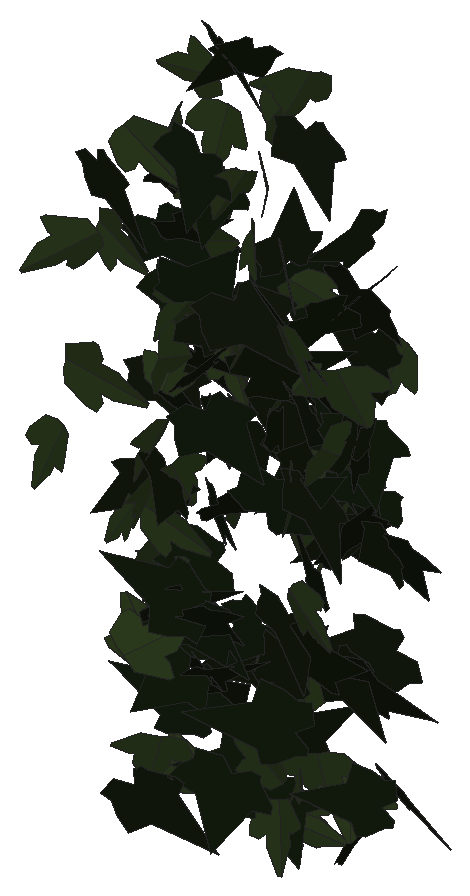
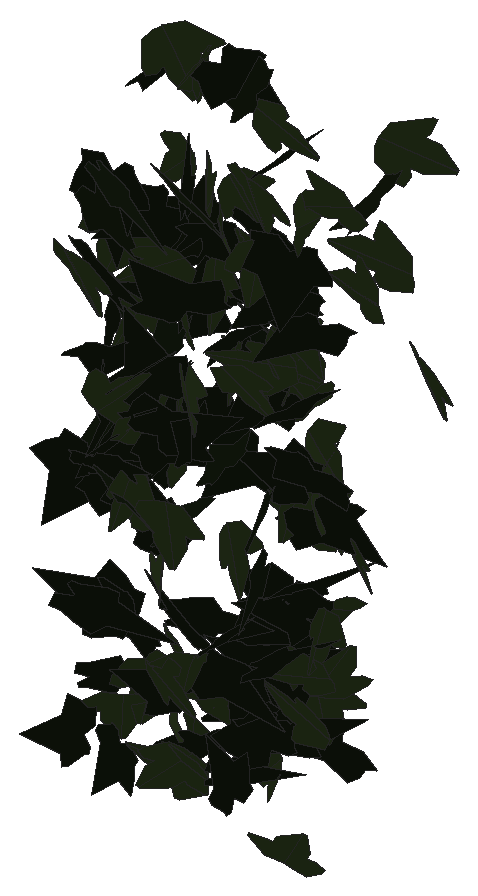
# SketchUp Ruby script. Lengths in inches.
U = 1.inch
M = Sketchup.active_model
def pt(a) = Geom::Point3d.new(a.map { |v| v * U })
def face(e, loops, mat)
  f = e.add_face(loops[0].map { |a| pt(a) })
  loops[1..].each { |l| e.add_face(l.map { |a| pt(a) }).erase! }
  f.material = f.back_material = mat if mat
  f
end
# faces: each face lists its corners as indices into pts; further lists are holes
def faces(e, pts, list, mat = nil) = list.each { |f| face(e, (f[0].is_a?(Array) ? f : [f]).map { |l| l.map { |i| pts[i] } }, mat) }
# xy, xz, yz: faces in a plane at the given z, y or x. An outline is a flat list of corners, or four numbers for a rectangle; further outlines are holes
def ring(l) = l.size == 4 ? [[l[0], l[1]], [l[2], l[1]], [l[2], l[3]], [l[0], l[3]]] : l.each_slice(2).to_a
def flat(e, list, mat, &to3) = list.each { |f| face(e, (f[0].is_a?(Array) ? f : [f]).map { |l| ring(l).map { |u, v| to3.(u, v) } }, mat) }
def xy(e, z, list, mat = nil) = flat(e, list, mat) { |x, y| [x, y, z] }
def xz(e, y, list, mat = nil) = flat(e, list, mat) { |x, z| [x, y, z] }
def yz(e, x, list, mat = nil) = flat(e, list, mat) { |y, z| [x, y, z] }
def lines(e, pts, list) = list.each { |a, b| e.add_line(pt(pts[a]), pt(pts[b])) }
# prism: a flat outline (further loops are holes) pulled along v
def prism(e, loops, v, mat = nil)
  f = face(e, loops, mat); d = Geom::Vector3d.new(v.map { |x| x * U })
  f.pushpull(f.normal.samedirection?(d) ? d.length : -d.length)
end
def box(e, o, s, mat = nil) = prism(e, [[o, [o[0] + s[0], o[1], o[2]], [o[0] + s[0], o[1] + s[1], o[2]], [o[0], o[1] + s[1], o[2]]]], [0, 0, s[2]], mat)
def at(x, y, z, deg = 0) = Geom::Transformation.translation(pt([x, y, z])) * Geom::Transformation.rotation(ORIGIN, Z_AXIS, deg.degrees)
def axes(o, x, y, z) = Geom::Transformation.new([*x, 0, *y, 0, *z, 0, *pt(o).to_a, 1])
def part(name) = M.definitions.add(name)
# library, detail: a bought-in or finely detailed component or shape, given as its bounding box
def library(name, o, s) = part(name).tap { |d| box(d.entities, o, s) }
def detail(e, o, s) = box(e.add_group.entities, o, s)
def put(e, d, t, mat = nil) = e.add_instance(d, t).tap { |i| i.material = mat if mat }
def group(e, t, mat = nil) = e.add_group.tap { |g| g.transformation = t; g.material = mat if mat }.entities
root = M.entities
M.materials.add("1026 AP 7946 SUNNY SIDE UP").color = [254, 231, 186]
M.materials.add("efeu1").color = [18, 25, 13]
M.materials.add("efeu2").color = [43, 57, 29]
c1 = part("ivyleaf_10")
p = [[0,0.5,-0.03],[-0.0625,2.02,-0.43],[-0.19,2.01,-0.46],[-0.54,1.05,-0.29],[-0.52,0.625,-0.18],[-0.83,0.76,-0.28],
  [-1.16,0.64,-0.33],[-1.15,0.33,-0.24],[-0.77,-0.39,0.02],[-0.3,-0.51,0.16],[0.04,-0.48,0.23],[-0.02,2.01,-0.4375],
  [-0.06,2.01,-0.43],[0.04,-0.49,0.23],[0.67,-0.49,0.14],[1.38,0.36,-0.2],[1.375,0.51,-0.24],[0.81,0.65,-0.19],
  [0.62,0.59,-0.15],[0.6,1.09,-0.28],[0.5,1.23,-0.31]]
faces(c1.entities,p,[[0,1,2,3,4,5,6,7,8,9,10],[11,12,0,13,14,15,16,17,18,19,20]],"efeu2")
c2 = part("ivyleaf_9")
p = [[1.54,2.16,1.25],[1.36,2.04,1.19],[-0.21,0.99,0.68],[-0.71,1.11,0.82],[-0.85,0.86,0.67],[-0.8,0.17,0.21],
  [-0.9,-0.01,0.1],[-0.67,-0.16,-0.02],[-0.08,-0.08,-0.05],[-0.03,-0.6,-0.4],[0.65,-0.88,-0.66],[0.83,-0.6,-0.49],
  [1.29,-0.42,-0.43],[1.8125,-0.07,-0.26],[1.21,0.44,0.15]]
faces(c2.entities,p,[[0,1,2,3,4,5,6,7,8,9,10,11,12,13,14]],"efeu1")
put(root,c1,axes([128.42,208.2,277.38],[-0.11981,-0.18538,0.35374],[-0.16586,-0.32816,-0.20792],[0.59225,-0.1294,0.01334]),"1026 AP 7946 SUNNY SIDE UP")
put(root,c1,axes([128.52,208.07,275.41],[0.02717,0.00224,0.40839],[0.62094,0.03465,-0.01773],[-0.05458,0.39527,0.00157]),"1026 AP 7946 SUNNY SIDE UP")
put(root,c1,axes([127.97,208.17,274.1],[0.44169,-0.27483,0.02712],[0.00539,-0.0363,-0.40434],[0.43433,0.27994,-0.02256]),"1026 AP 7946 SUNNY SIDE UP")
put(root,c1,axes([131.47,209,276.5],[-0.30463,0.20215,-0.19161],[0.17913,-0.14952,-0.28875],[-0.39439,-0.22405,0.01685]),"1026 AP 7946 SUNNY SIDE UP")
put(root,c2,axes([128.72,209.08,268.42],[0.0398,-0.10331,-0.35879],[0.46844,0.20474,-0.03913],[0.32534,-0.28215,0.10024]),"1026 AP 7946 SUNNY SIDE UP")
put(root,c1,axes([128.98,209.22,269.13],[-0.37267,-0.23168,0.04947],[-0.02963,-0.05113,-0.34091],[0.37129,-0.23663,0.02245]),"1026 AP 7946 SUNNY SIDE UP")
put(root,c1,axes([131.36,209.375,272.16],[-0.19428,0.10101,-0.33264],[0.32312,-0.25144,-0.16322],[-0.4237,-0.23807,0.02805]),"1026 AP 7946 SUNNY SIDE UP")
put(root,c1,axes([128.6,209.1875,270.54],[0.31198,0.0225,-0.31751],[0.3079,0.27435,0.15205],[0.37616,-0.24323,0.13888]),"1026 AP 7946 SUNNY SIDE UP")
put(root,c2,axes([129.91,209.64,268.76],[-0.31064,-0.30865,-0.02061],[0.04185,0.0046,-0.37694],[0.48436,-0.19835,0.01935]),"1026 AP 7946 SUNNY SIDE UP")
put(root,c2,axes([130.95,209.66,269.84],[-0.35005,0.0129,0.30611],[-0.46477,-0.05002,-0.22625],[0.05093,-0.36784,0.03931]),"1026 AP 7946 SUNNY SIDE UP")
put(root,c2,axes([128.98,209.82,270.02],[-0.31738,-0.20262,0.15102],[-0.12374,-0.1289,-0.29362],[0.37439,-0.21437,0.03098]),"1026 AP 7946 SUNNY SIDE UP")
put(root,c2,axes([129.61,209.51,274.45],[0.01083,-0.23233,-0.30337],[0.01332,0.29323,-0.23749],[0.58802,-0.00236,0.01097]),"1026 AP 7946 SUNNY SIDE UP")
put(root,c2,axes([130.75,209.86,271.48],[0.05918,-0.3586,0.16433],[0.0429,-0.15952,-0.37226],[0.61695,0.04549,0.01012]),"1026 AP 7946 SUNNY SIDE UP")
put(root,c1,axes([130.61,209.76,268.36],[0.44483,-0.13392,0.22782],[0.28607,-0.13135,-0.32138],[0.29027,0.33469,-0.0324]),"1026 AP 7946 SUNNY SIDE UP")
put(root,c2,axes([127.52,209.74,277.54],[0.29023,-0.33567,-0.03726],[-0.04253,0.0242,-0.39431],[0.52885,0.18616,-0.01127]),"1026 AP 7946 SUNNY SIDE UP")
put(root,c2,axes([128.56,209.9375,272.9],[-0.02994,-0.24284,0.25414],[-0.02519,-0.24756,-0.25238],[0.54528,-0.02477,0.0023]),"1026 AP 7946 SUNNY SIDE UP")
put(root,c2,axes([131.14,209.77,271.01],[0.06651,-0.0184,0.34077],[0.33948,-0.25154,-0.04431],[0.39534,0.21909,-0.01928]),"1026 AP 7946 SUNNY SIDE UP")
put(root,c2,axes([130.47,209.92,276.11],[0.25901,-0.25402,0.27156],[0.17644,-0.24175,-0.31196],[0.54963,0.19732,-0.02782]),"1026 AP 7946 SUNNY SIDE UP")
put(root,c1,axes([131.83,209.72,275.6875],[-0.48263,-0.23109,-0.12927],[0.1829,0.05141,-0.39449],[0.36973,-0.32708,0.0264]),"1026 AP 7946 SUNNY SIDE UP")
put(root,c2,axes([128.92,209.98,270.99],[-0.18236,-0.36285,-0.08835],[-0.05779,-0.07608,0.39181],[-0.58267,0.12111,-0.01121]),"1026 AP 7946 SUNNY SIDE UP")
put(root,c2,axes([131.43,209.6875,272.125],[0.03109,-0.12438,0.31495],[-0.08241,0.30192,0.1315],[-0.51343,-0.05599,-0.00203]),"1026 AP 7946 SUNNY SIDE UP")
put(root,c1,axes([128.37,209.89,272.25],[0.0374,0.00642,0.39893],[0.60537,-0.04221,-0.02389],[0.06564,0.38563,-0.00697]),"1026 AP 7946 SUNNY SIDE UP")
put(root,c1,axes([128.37,209.97,273.56],[0.06061,-0.34943,0.14222],[0.03445,-0.13845,-0.36292],[0.59092,0.04391,0.00657]),"1026 AP 7946 SUNNY SIDE UP")
put(root,c2,axes([131.04,210.02,273.5],[0.13433,-0.39367,0.03087],[-0.00202,-0.03323,-0.4151],[0.62108,0.08504,-0.00802]),"1026 AP 7946 SUNNY SIDE UP")
put(root,c2,axes([130.51,209.76,273.13],[-0.156,0.06215,0.34462],[0.5213,-0.05907,0.11237],[0.11785,0.34354,-0.04089]),"1026 AP 7946 SUNNY SIDE UP")
put(root,c2,axes([129.91,209.8125,276.16],[0.00295,-0.22583,-0.33937],[0.23158,0.30529,-0.21379],[0.58197,-0.12033,0.08679]),"1026 AP 7946 SUNNY SIDE UP")
put(root,c1,axes([129.15,209.97,268.36],[-0.23781,0.24366,-0.22268],[0.15602,-0.19412,-0.29621],[-0.48934,-0.18031,0.01378]),"1026 AP 7946 SUNNY SIDE UP")
put(root,c1,axes([128.28,209.96,272.72],[0.06747,-0.3707,0.04766],[0.0016,-0.04857,-0.3847],[0.58783,0.04268,-0.00442]),"1026 AP 7946 SUNNY SIDE UP")
put(root,c1,axes([127.86,209.9,272.16],[0.29968,-0.24874,-0.05957],[-0.07734,0.03326,-0.32206],[0.39352,0.19596,-0.01793]),"1026 AP 7946 SUNNY SIDE UP")
put(root,c1,axes([131.58,209.67,274.51],[-0.1065,-0.24369,-0.32412],[0.16029,0.29642,-0.25855],[0.6031,-0.12181,0.01148]),"1026 AP 7946 SUNNY SIDE UP")
put(root,c2,axes([130.55,210.12,276.57],[-0.06709,0.04271,0.32963],[-0.03227,-0.32221,0.03963],[0.50617,-0.01488,0.04621]),"1026 AP 7946 SUNNY SIDE UP")
put(root,c1,axes([130.43,209.84,268.97],[-0.31407,0.0873,-0.30188],[-0.38511,0.16483,0.22316],[0.28905,0.31446,-0.03068]),"1026 AP 7946 SUNNY SIDE UP")
put(root,c2,axes([129.02,209.79,270.9],[0.39646,0.18566,0.07963],[0.116,0.02812,-0.32171],[-0.29349,0.26191,-0.01959]),"1026 AP 7946 SUNNY SIDE UP")
put(root,c2,axes([131.96,209.72,274.51],[0.02494,0.19172,0.28427],[-0.0728,0.27377,-0.19238],[-0.52187,-0.02903,0.04042]),"1026 AP 7946 SUNNY SIDE UP")
put(root,c2,axes([128.85,210.28,277.91],[-0.08492,-0.36305,0.16181],[-0.04475,-0.15664,-0.37902],[0.62169,-0.06086,-0.00518]),"1026 AP 7946 SUNNY SIDE UP")
put(root,c1,axes([127.32,210.14,276.25],[0.07164,-0.00691,0.3717],[0.54256,-0.10579,-0.04759],[0.16637,0.34798,-0.00486]),"1026 AP 7946 SUNNY SIDE UP")
put(root,c2,axes([129.61,209.8,272.9],[0.25531,0.23186,0.16524],[0.15503,0.12509,-0.29076],[-0.41407,0.1898,-0.00697]),"1026 AP 7946 SUNNY SIDE UP")
put(root,c1,axes([130.82,209.84,273.43],[0.10121,-0.21071,-0.34123],[-0.04697,0.33085,-0.22167],[0.6139,0.06005,0.0393]),"1026 AP 7946 SUNNY SIDE UP")
put(root,c2,axes([132.04,210.24,268.78],[-0.25759,-0.02385,0.27858],[-0.39344,-0.10962,-0.16668],[0.16608,-0.29668,0.0372]),"1026 AP 7946 SUNNY SIDE UP")
put(root,c2,axes([128.83,210,274.47],[0.13185,0.30143,0.07099],[-0.04864,-0.06108,0.32168],[0.48316,-0.08841,0.01301]),"1026 AP 7946 SUNNY SIDE UP")
put(root,c2,axes([130.25,210.16,268.44],[-0.11094,-0.29457,-0.15821],[0.0837,0.14322,-0.31075],[0.51438,-0.08684,0.01644]),"1026 AP 7946 SUNNY SIDE UP")
put(root,c2,axes([128.2,210.23,272.65],[0.05694,0.06394,-0.33216],[-0.16625,-0.30526,-0.0763],[-0.48999,0.111,-0.01271]),"1026 AP 7946 SUNNY SIDE UP")
put(root,c2,axes([128.91,209.96,269.75],[0.21284,0.26955,-0.12498],[0.06576,0.11632,0.3111],[0.46112,-0.14101,0.01332]),"1026 AP 7946 SUNNY SIDE UP")
put(root,c2,axes([128.74,210.08,270.77],[-0.09104,-0.11814,-0.3254],[0.308,0.24827,-0.13148],[0.43044,-0.20264,0.02525]),"1026 AP 7946 SUNNY SIDE UP")
put(root,c2,axes([128.39,209.93,270.82],[0.12708,0.22605,-0.22191],[0.06301,0.21449,0.24715],[0.48832,-0.0865,0.02586]),"1026 AP 7946 SUNNY SIDE UP")
put(root,c1,axes([130.05,210.05,275.62],[-0.0313,-0.33319,-0.18832],[0.03506,0.17982,-0.34265],[0.59512,-0.02812,0.01028]),"1026 AP 7946 SUNNY SIDE UP")
put(root,c2,axes([131.875,209.99,274.52],[0.10229,-0.08754,-0.32671],[-0.38917,0.19919,-0.10795],[0.33967,0.25458,-0.0253]),"1026 AP 7946 SUNNY SIDE UP")
put(root,c2,axes([130.12,209.93,275.04],[0.1016,0.06476,0.40098],[0.57149,0.14282,-0.08588],[-0.24006,0.36741,-0.03475]),"1026 AP 7946 SUNNY SIDE UP")
put(root,c1,axes([128.13,210.15,269.94],[0.27018,0.34267,0.0829],[-0.0884,-0.05949,0.39384],[0.54566,-0.17931,0.02276]),"1026 AP 7946 SUNNY SIDE UP")
put(root,c1,axes([130.5,210.42,268.77],[0.0479,0.00333,0.37118],[0.36567,-0.27634,-0.01924],[0.43271,0.23316,-0.02483]),"1026 AP 7946 SUNNY SIDE UP")
put(root,c1,axes([128.47,209.94,274.78],[0.00729,-0.16399,-0.36684],[0.10398,0.3504,-0.16374],[0.60626,-0.05812,0.03249]),"1026 AP 7946 SUNNY SIDE UP")
put(root,c1,axes([128.54,210.1,272.92],[-0.23008,-0.3178,-0.18229],[0.12304,0.15677,-0.35948],[0.55715,-0.16586,0.00411]),"1026 AP 7946 SUNNY SIDE UP")
put(root,c1,axes([131.05,210.1875,269.15],[-0.44421,-0.20526,-0.05946],[0.09776,0.01034,-0.35854],[0.32019,-0.28793,0.02698]),"1026 AP 7946 SUNNY SIDE UP")
put(root,c2,axes([131.05,209.98,276.28],[-0.01642,0.09272,-0.32589],[-0.03758,0.31598,0.09791],[0.51777,0.02587,-0.00323]),"1026 AP 7946 SUNNY SIDE UP")
put(root,c2,axes([128.6,210.16,270.13],[-0.40939,-0.1863,0.17155],[0.18492,0.12254,0.3293],[-0.34793,0.28435,-0.02683]),"1026 AP 7946 SUNNY SIDE UP")
put(root,c2,axes([130.67,210.37,278.86],[0.03706,-0.36571,-0.05224],[-0.01671,0.04804,-0.37717],[0.57986,0.02476,-0.00753]),"1026 AP 7946 SUNNY SIDE UP")
put(root,c2,axes([130.62,210.52,274.39],[-0.05142,-0.19229,0.31216],[0.05578,-0.30559,-0.19693],[0.56299,0.01271,0.04802]),"1026 AP 7946 SUNNY SIDE UP")
put(root,c1,axes([130.29,210.35,267.94],[-0.01379,-0.05495,-0.36266],[0.53027,-0.11398,0.00901],[-0.1793,-0.33286,0.05456]),"1026 AP 7946 SUNNY SIDE UP")
put(root,c2,axes([128.8,210.24,275.68],[-0.29144,0.01598,0.27227],[0.40521,-0.06269,0.18978],[0.09495,0.31658,0.02577]),"1026 AP 7946 SUNNY SIDE UP")
put(root,c2,axes([128.82,210.41,269.05],[-0.07579,0.05465,0.37309],[-0.57498,-0.02124,-0.047],[0.02215,-0.36442,0.0565]),"1026 AP 7946 SUNNY SIDE UP")
put(root,c2,axes([129.22,210.32,275.39],[-0.41583,0.18301,0.04526],[-0.07935,0.0022,-0.33016],[-0.28472,-0.2679,0.02591]),"1026 AP 7946 SUNNY SIDE UP")
put(root,c2,axes([128.33,210.55,269.84],[0.14168,-0.15404,0.29092],[0.17816,-0.26024,-0.18443],[0.47467,0.14365,-0.01761]),"1026 AP 7946 SUNNY SIDE UP")
put(root,c1,axes([128.33,210.17,274.27],[0.16321,0.22401,-0.20862],[0.11129,0.1915,0.25513],[0.46298,-0.125,0.01221]),"1026 AP 7946 SUNNY SIDE UP")
put(root,c1,axes([127.58,210.41,277.71],[0.27751,0.05725,0.3029],[0.4664,0.01145,-0.18585],[-0.06199,0.34245,-0.04236]),"1026 AP 7946 SUNNY SIDE UP")
put(root,c2,axes([131.8125,210.7,272.6],[-0.16876,-0.11996,0.34103],[-0.04902,-0.34215,-0.13986],[0.55248,-0.067,0.09176]),"1026 AP 7946 SUNNY SIDE UP")
put(root,c1,axes([129.47,210.61,276.68],[0.12425,-0.0496,0.32143],[0.35128,-0.21905,-0.09535],[0.35187,0.23619,-0.01831]),"1026 AP 7946 SUNNY SIDE UP")
put(root,c1,axes([131.36,210.44,268.72],[0.39697,0.23813,-0.00839],[0.01473,-0.02374,-0.35683],[-0.37445,0.25152,-0.02293]),"1026 AP 7946 SUNNY SIDE UP")
put(root,c2,axes([131.63,210.34,276.74],[0.42375,0.00599,-0.31533],[-0.47967,-0.0298,-0.27743],[-0.04138,0.40676,-0.01329]),"1026 AP 7946 SUNNY SIDE UP")
put(root,c1,axes([128.43,210.64,275.44],[-0.06936,-0.31256,0.22853],[-0.03706,-0.22245,-0.32643],[0.60316,-0.04961,0.00622]),"1026 AP 7946 SUNNY SIDE UP")
put(root,c1,axes([130.4,210.4,268.12],[-0.36028,-0.09095,-0.19683],[0.29491,0.04148,-0.25249],[0.15249,-0.2951,0.02325]),"1026 AP 7946 SUNNY SIDE UP")
put(root,c2,axes([130.11,210.4,270.04],[-0.2167,0.26675,0.22953],[0.19414,-0.18473,0.30754],[0.50922,0.18394,-0.01958]),"1026 AP 7946 SUNNY SIDE UP")
put(root,c2,axes([129.51,210.64,268.32],[-0.25889,-0.0582,0.25785],[-0.35416,-0.11122,-0.17969],[0.19555,-0.27848,0.01592]),"1026 AP 7946 SUNNY SIDE UP")
put(root,c1,axes([130.48,210.35,274.9],[0.38344,-0.11141,0.22985],[-0.27498,0.14729,0.27277],[-0.2808,-0.29637,0.04675]),"1026 AP 7946 SUNNY SIDE UP")
put(root,c1,axes([129.03,210.66,274.72],[0.35902,-0.07211,0.27239],[0.37836,-0.1131,-0.24612],[0.20758,0.33086,-0.02252]),"1026 AP 7946 SUNNY SIDE UP")
put(root,c2,axes([131.43,210.21,272.84],[-0.10982,0.12725,-0.38525],[-0.24347,0.34135,0.15116],[0.57259,0.16955,-0.00961]),"1026 AP 7946 SUNNY SIDE UP")
put(root,c1,axes([130.41,210.55,270.03],[0.28855,-0.24546,-0.06906],[-0.08299,0.04237,-0.31502],[0.39081,0.19023,-0.01591]),"1026 AP 7946 SUNNY SIDE UP")
put(root,c1,axes([129.23,210.65,277.53],[-0.12321,-0.29407,0.1178],[-0.0347,-0.11415,-0.31409],[0.49587,-0.08105,0.00729]),"1026 AP 7946 SUNNY SIDE UP")
put(root,c1,axes([130.08,210.28,278.98],[0.06068,-0.01037,-0.3658],[0.06242,0.355,-0.00416],[0.55498,-0.0388,0.04046]),"1026 AP 7946 SUNNY SIDE UP")
put(root,c2,axes([131.39,210.68,274.29],[-0.18791,-0.29959,-0.13173],[0.11934,0.10499,-0.33028],[0.49701,-0.13848,0.0295]),"1026 AP 7946 SUNNY SIDE UP")
put(root,c2,axes([130.38,210.34,276.84],[-0.44213,0.18397,-0.12605],[-0.13985,0.08887,0.34579],[0.31901,0.29393,-0.02311]),"1026 AP 7946 SUNNY SIDE UP")
put(root,c2,axes([129.45,210.84,270.47],[-0.14416,-0.22166,0.194],[-0.10009,-0.17873,-0.24804],[0.44757,-0.11136,0.00702]),"1026 AP 7946 SUNNY SIDE UP")
put(root,c1,axes([128.68,210.69,276.34],[-0.30359,0.04548,0.26312],[0.38677,-0.06806,0.20385],[0.12836,0.31264,0.00805]),"1026 AP 7946 SUNNY SIDE UP")
put(root,c1,axes([130.33,210.71,279.43],[-0.29391,-0.33558,0.12065],[-0.06333,-0.11363,-0.39589],[0.55627,-0.19024,0.01867]),"1026 AP 7946 SUNNY SIDE UP")
put(root,c2,axes([130.4,210.43,269.18],[-0.01466,0.02473,0.32534],[0.43799,0.15079,-0.00281],[-0.23671,0.27747,-0.02535]),"1026 AP 7946 SUNNY SIDE UP")
put(root,c2,axes([128.64,210.71,269.1],[0.54139,-0.03781,-0.07215],[0.11856,0.05829,0.35086],[-0.03914,-0.34645,0.0648]),"1026 AP 7946 SUNNY SIDE UP")
put(root,c2,axes([131.24,210.72,270.26],[0.25528,-0.11276,0.31292],[0.3764,-0.18828,-0.20449],[0.34474,0.28907,-0.00846]),"1026 AP 7946 SUNNY SIDE UP")
put(root,c2,axes([128.6,210.57,274.56],[0.50625,-0.00575,-0.01922],[-0.02995,-0.02716,-0.33069],[0.00653,0.32135,-0.02639]),"1026 AP 7946 SUNNY SIDE UP")
put(root,c1,axes([129.37,210.5,274.84],[-0.20577,0.2026,0.24049],[-0.22141,0.18519,-0.24704],[-0.43113,-0.1918,0.01209]),"1026 AP 7946 SUNNY SIDE UP")
put(root,c2,axes([130.36,210.89,273.42],[-0.04675,0.06939,-0.35839],[0.1491,-0.33526,-0.07911],[-0.53812,-0.09892,0.00921]),"1026 AP 7946 SUNNY SIDE UP")
put(root,c2,axes([130.91,210.8,270.39],[-0.09701,-0.06465,-0.3619],[0.55326,0.04822,-0.07259],[0.09333,-0.35303,0.05419]),"1026 AP 7946 SUNNY SIDE UP")
put(root,c2,axes([128.7,210.85,277.23],[-0.39796,-0.09036,-0.17694],[0.2784,0.00605,-0.27284],[0.12321,-0.30552,0.04498]),"1026 AP 7946 SUNNY SIDE UP")
put(root,c2,axes([131.4375,210.45,268.01],[-0.11745,0.10167,-0.33337],[-0.31241,0.25617,0.13143],[0.43335,0.21224,0.0044]),"1026 AP 7946 SUNNY SIDE UP")
put(root,c2,axes([129.28,210.86,279.49],[-0.07347,0.13698,-0.30012],[-0.00991,-0.29548,-0.14343],[-0.50719,-0.01407,0.04627]),"1026 AP 7946 SUNNY SIDE UP")
put(root,c2,axes([129.61,210.77,270.03],[0.05445,-0.00027,-0.34894],[-0.43261,-0.19861,-0.02998],[-0.31063,0.27655,-0.01942]),"1026 AP 7946 SUNNY SIDE UP")
put(root,c2,axes([128,210.8,273.45],[0.23606,-0.11232,0.24296],[0.29973,-0.13996,-0.19397],[0.28217,0.24264,0.00278]),"1026 AP 7946 SUNNY SIDE UP")
put(root,c1,axes([129.5,210.91,277.375],[-0.15433,0.14794,0.2892],[0.30405,-0.204,0.17974],[0.39414,0.2153,-0.02542]),"1026 AP 7946 SUNNY SIDE UP")
put(root,c1,axes([127.73,210.61,271.28],[-0.03233,-0.2707,-0.22453],[0.06958,0.21297,-0.27753],[0.5405,-0.04361,0.02229]),"1026 AP 7946 SUNNY SIDE UP")
put(root,c2,axes([131.55,210.77,276.62],[-0.20377,0.25377,-0.13591],[0.0662,-0.12792,-0.29366],[-0.44589,-0.13496,0.01851]),"1026 AP 7946 SUNNY SIDE UP")
put(root,c2,axes([131.83,210.63,275.47],[-0.33411,0.02692,-0.32098],[-0.48732,0.03362,0.22082],[0.06753,0.37575,0.00546]),"1026 AP 7946 SUNNY SIDE UP")
put(root,c2,axes([128.98,210.85,275.48],[0.08353,-0.32057,-0.11904],[-0.02433,0.11272,-0.33408],[0.5343,0.05525,0.0034]),"1026 AP 7946 SUNNY SIDE UP")
put(root,c2,axes([131.16,210.97,272.51],[-0.02239,0.0604,-0.31987],[-0.09385,-0.30609,-0.06025],[-0.48898,0.05598,0.02621]),"1026 AP 7946 SUNNY SIDE UP")
put(root,c1,axes([131.85,210.89,275.57],[0.51877,-0.20323,-0.03766],[-0.06865,-0.00352,-0.39833],[0.31703,0.3318,-0.02462]),"1026 AP 7946 SUNNY SIDE UP")
put(root,c2,axes([128.66,210.98,279.33],[0.24347,-0.25196,0.1317],[0.07317,-0.12269,-0.3045],[0.43923,0.1601,-0.02228]),"1026 AP 7946 SUNNY SIDE UP")
put(root,c1,axes([128.57,210.8125,278.89],[-0.12084,0.04698,0.32095],[-0.49495,-0.00736,-0.07896],[-0.00634,-0.32054,0.04694]),"1026 AP 7946 SUNNY SIDE UP")
put(root,c2,axes([130.29,211.02,274.18],[0.54486,-0.10261,-0.128],[0.20314,0.00309,0.37031],[-0.15025,-0.36791,0.03649]),"1026 AP 7946 SUNNY SIDE UP")
put(root,c2,axes([129.1,211.09,273.4375],[0.04035,-0.26447,0.19508],[0.06688,-0.1871,-0.27408],[0.50846,0.0456,0.02057]),"1026 AP 7946 SUNNY SIDE UP")
put(root,c1,axes([129.83,210.88,270.09],[0.29483,0.23124,0.01784],[0.03828,0.00082,-0.30611],[-0.36246,0.18818,-0.01782]),"1026 AP 7946 SUNNY SIDE UP")
put(root,c2,axes([130.625,211.17,274.32],[-0.13177,-0.27956,0.17396],[-0.03631,-0.17046,-0.30071],[0.51356,-0.08378,0.02337]),"1026 AP 7946 SUNNY SIDE UP")
put(root,c1,axes([128.1875,210.86,267.58],[0.46104,0.06634,0.10259],[-0.16453,0.01634,0.30743],[0.09024,-0.3091,0.03638]),"1026 AP 7946 SUNNY SIDE UP")
put(root,c2,axes([127.65,210.98,273.83],[-0.17769,-0.14492,-0.29732],[0.42286,0.12556,-0.1732],[0.27908,-0.28253,0.07312]),"1026 AP 7946 SUNNY SIDE UP")
put(root,c1,axes([127.6,211.02,269.87],[0.14665,-0.10131,-0.33302],[0.44073,-0.16416,0.1356],[-0.29761,-0.29304,0.03671]),"1026 AP 7946 SUNNY SIDE UP")
put(root,c1,axes([130.22,210.85,276.1],[-0.26088,-0.10033,-0.2493],[0.37419,0.06045,-0.194],[0.17023,-0.28663,0.04439]),"1026 AP 7946 SUNNY SIDE UP")
put(root,c2,axes([128.09,210.77,276.39],[0.3977,0.1618,0.10278],[0.15752,0.02588,-0.30756],[-0.25313,0.27032,-0.02991]),"1026 AP 7946 SUNNY SIDE UP")
put(root,c1,axes([130.18,211.18,271.27],[-0.01543,-0.04473,-0.30463],[0.07367,-0.29218,0.04226],[-0.46405,-0.0449,0.01684]),"1026 AP 7946 SUNNY SIDE UP")
put(root,c1,axes([130.74,211.04,273.37],[0.06345,0.30687,0.17121],[-0.0536,-0.16127,0.3177],[0.54481,-0.0516,0.01132]),"1026 AP 7946 SUNNY SIDE UP")
put(root,c1,axes([127.66,210.9,270.61],[0.1203,0.07277,0.29016],[0.40426,0.11846,-0.10293],[-0.2127,0.26631,-0.03152]),"1026 AP 7946 SUNNY SIDE UP")
put(root,c1,axes([129.9,210.9,274.43],[0.07456,-0.30573,-0.16672],[-0.06978,0.15486,-0.31729],[0.53815,0.06244,-0.01804]),"1026 AP 7946 SUNNY SIDE UP")
put(root,c2,axes([131.63,210.89,272.52],[0.53704,0.0438,-0.08734],[-0.1248,-0.04617,-0.3532],[-0.08392,0.34892,-0.03367]),"1026 AP 7946 SUNNY SIDE UP")
put(root,c1,axes([127.72,211.2,277.71],[-0.0604,0.09388,-0.30843],[-0.04498,-0.30194,-0.09536],[-0.49211,0.01608,0.04657]),"1026 AP 7946 SUNNY SIDE UP")
put(root,c2,axes([130.89,211.0625,273.3],[0.10464,-0.31312,-0.08813],[-0.01917,0.08304,-0.32925],[0.5093,0.06746,0.00572]),"1026 AP 7946 SUNNY SIDE UP")
put(root,c1,axes([128.3,210.93,275.21],[-0.02688,-0.05737,-0.34721],[0.52795,0.05902,-0.02758],[0.09852,-0.33193,0.05305]),"1026 AP 7946 SUNNY SIDE UP")
put(root,c2,axes([131.17,210.99,272.52],[-0.34549,0.22828,-0.00654],[-0.01629,-0.02056,-0.32577],[-0.35878,-0.21889,0.02109]),"1026 AP 7946 SUNNY SIDE UP")
put(root,c1,axes([131.07,211.12,273.75],[-0.36122,-0.07849,-0.21621],[-0.32387,-0.04274,0.24901],[-0.13704,0.30791,-0.0186]),"1026 AP 7946 SUNNY SIDE UP")
put(root,c2,axes([130.22,211.0625,273.53],[0.0467,0.03267,0.36927],[-0.54016,0.10932,0.01971],[-0.16797,-0.34247,0.03929]),"1026 AP 7946 SUNNY SIDE UP")
put(root,c2,axes([131.23,211.02,277.16],[-0.36872,0.27034,-0.02153],[-0.00814,-0.03412,-0.36788],[-0.42646,-0.23309,0.02564]),"1026 AP 7946 SUNNY SIDE UP")
put(root,c2,axes([129.78,210.88,273.48],[-0.0692,-0.0667,0.31956],[0.24201,0.2698,0.08374],[-0.43693,0.16,-0.00423]),"1026 AP 7946 SUNNY SIDE UP")
put(root,c1,axes([128.97,211.07,272.35],[-0.00046,-0.36884,-0.06801],[0.00331,0.06392,-0.3796],[0.5886,-0.00065,0.00208]),"1026 AP 7946 SUNNY SIDE UP")
put(root,c1,axes([128.51,211.18,278.01],[0.53751,-0.17267,0.07512],[0.0842,-0.05748,-0.39392],[0.28307,0.34498,-0.02546]),"1026 AP 7946 SUNNY SIDE UP")
put(root,c2,axes([127.5625,211,276.1],[0.01289,-0.16999,-0.29294],[0.12034,0.27674,-0.16712],[0.50549,-0.06155,0.04726]),"1026 AP 7946 SUNNY SIDE UP")
put(root,c1,axes([130.14,211.08,272.3125],[-0.51883,0.03418,0.09103],[-0.14278,-0.02521,-0.34016],[-0.0415,-0.3406,0.03229]),"1026 AP 7946 SUNNY SIDE UP")
put(root,c2,axes([131.5,211.22,270.61],[-0.08278,-0.09228,-0.34989],[-0.39322,-0.23109,0.10342],[-0.38827,0.2537,-0.03015]),"1026 AP 7946 SUNNY SIDE UP")
put(root,c2,axes([128.48,211.03,272.02],[0.29715,-0.13806,-0.22535],[-0.30355,0.10359,-0.23942],[0.26916,0.26924,-0.02122]),"1026 AP 7946 SUNNY SIDE UP")
put(root,c2,axes([128.05,211.01,277.06],[0.31757,0.25788,-0.10497],[-0.08189,-0.09037,-0.33766],[-0.4291,0.2081,-0.01324]),"1026 AP 7946 SUNNY SIDE UP")
put(root,c2,axes([131.47,211.22,268.51],[0.36005,-0.19851,0.12229],[0.11412,-0.0986,-0.31171],[0.34629,0.2389,-0.02443]),"1026 AP 7946 SUNNY SIDE UP")
put(root,c2,axes([127.75,211.375,274.93],[-0.14748,-0.3428,0.08846],[-0.01988,-0.08754,-0.36648],[0.55608,-0.09405,0.01036]),"1026 AP 7946 SUNNY SIDE UP")
put(root,c1,axes([130.77,211.04,272.57],[-0.10358,-0.27324,-0.17728],[0.11763,0.15633,-0.28689],[0.49261,-0.09478,0.03123]),"1026 AP 7946 SUNNY SIDE UP")
put(root,c1,axes([130.29,211.01,269.82],[0.13287,-0.0934,-0.33354],[-0.3593,0.2287,-0.12828],[0.38833,0.24356,-0.00457]),"1026 AP 7946 SUNNY SIDE UP")
put(root,c2,axes([128.21,211.4,270.79],[-0.01249,-0.27471,-0.20627],[-0.00997,-0.19857,0.28196],[-0.53299,0.01015,-0.00044]),"1026 AP 7946 SUNNY SIDE UP")
put(root,c2,axes([128.73,211.36,268.6],[0.03043,-0.10289,0.32554],[0.15731,-0.30066,-0.10873],[0.49923,0.10101,0.01442]),"1026 AP 7946 SUNNY SIDE UP")
put(root,c1,axes([128.86,211.17,274.95],[0.37321,-0.07583,-0.20617],[-0.30908,0.0393,-0.25583],[0.13146,0.30768,-0.01619]),"1026 AP 7946 SUNNY SIDE UP")
put(root,c2,axes([131.13,211.31,272.95],[-0.43025,-0.12818,-0.02244],[0.04713,-0.01454,-0.31023],[0.19875,-0.27405,0.02499]),"1026 AP 7946 SUNNY SIDE UP")
put(root,c2,axes([129.8125,211.04,275.625],[-0.2899,0.00233,0.32818],[0.49099,0.07418,0.18606],[-0.09915,0.3605,-0.0382]),"1026 AP 7946 SUNNY SIDE UP")
put(root,c2,axes([128.2,211.46,273.03],[0.16301,-0.12973,-0.31846],[0.3755,-0.19743,0.16711],[-0.36846,-0.2586,0.02941]),"1026 AP 7946 SUNNY SIDE UP")
put(root,c1,axes([128.43,211.16,276.99],[-0.30377,-0.27824,-0.08718],[0.0873,0.0625,-0.34845],[0.44815,-0.20078,0.00879]),"1026 AP 7946 SUNNY SIDE UP")
